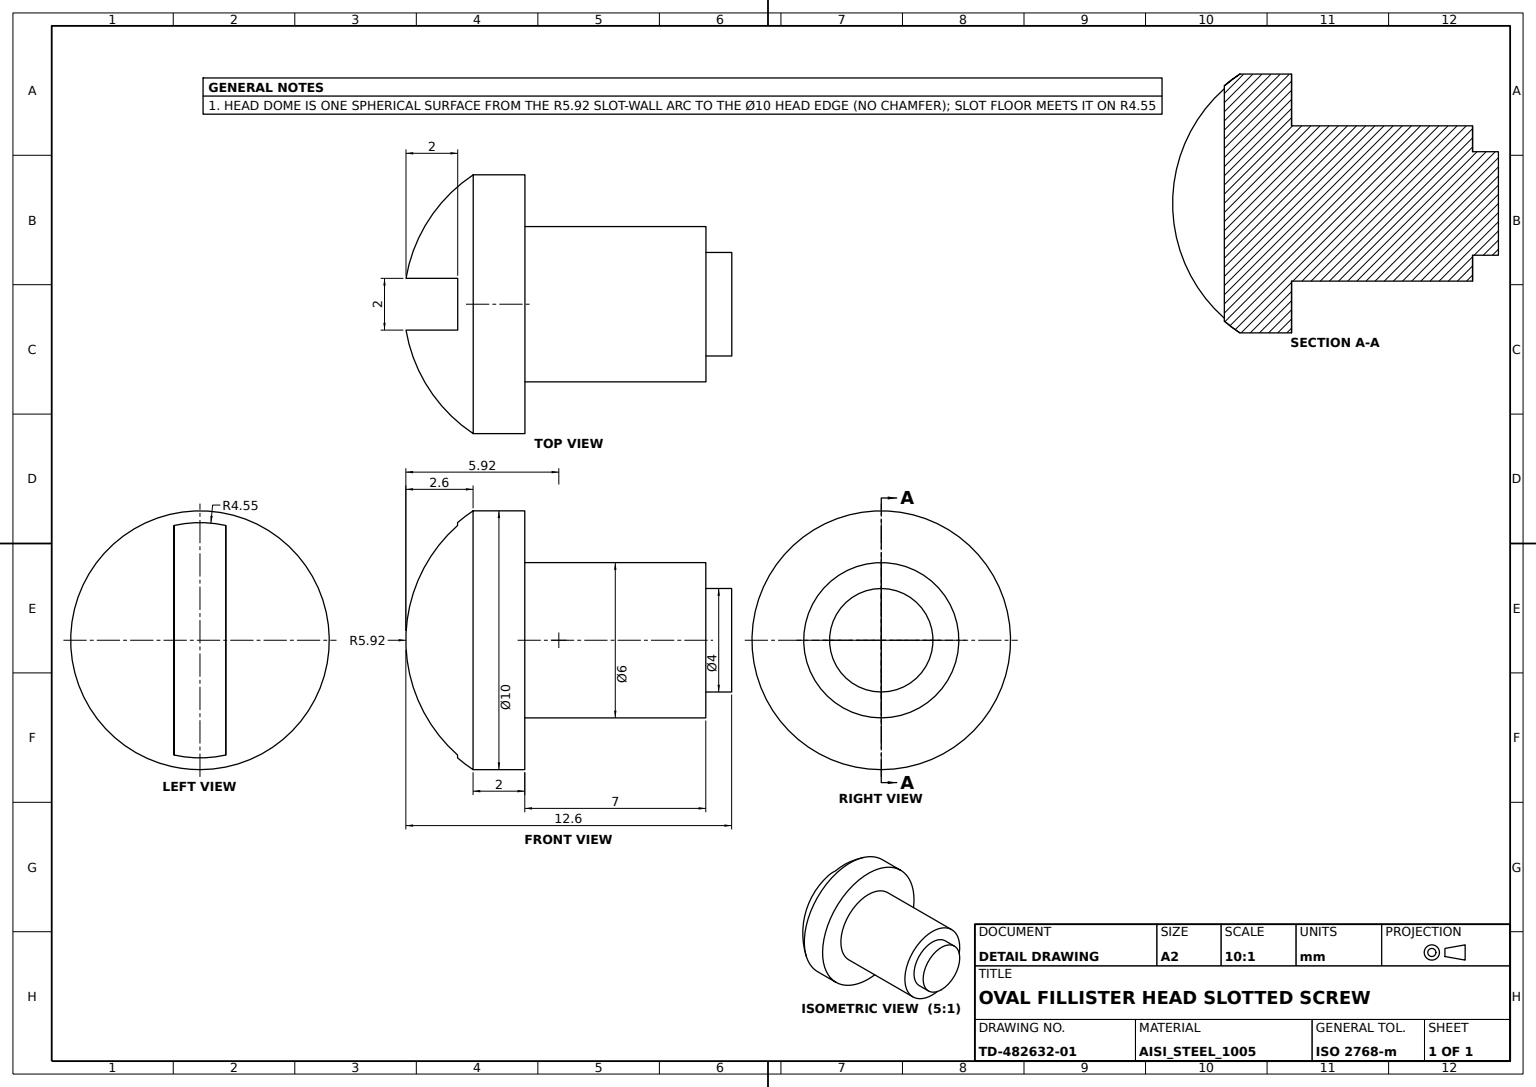
ISO-10303-21;
HEADER;
FILE_DESCRIPTION((''),'2;1');
FILE_NAME('','',(''),(''),'','','');
FILE_SCHEMA(('AUTOMOTIVE_DESIGN'));
ENDSEC;
DATA;
#1=APPLICATION_CONTEXT('');
#2=PRODUCT_CONTEXT('',#1,'mechanical');
#3=PRODUCT('','','',(#2));
#4=PRODUCT_DEFINITION_FORMATION('','',#3);
#5=PRODUCT_DEFINITION_CONTEXT('',#1,'design');
#6=PRODUCT_DEFINITION('','',#4,#5);
#7=PRODUCT_DEFINITION_SHAPE('','',#6);
#8=(LENGTH_UNIT()NAMED_UNIT(*)SI_UNIT(.MILLI.,.METRE.));
#9=(NAMED_UNIT(*)PLANE_ANGLE_UNIT()SI_UNIT($,.RADIAN.));
#10=(NAMED_UNIT(*)SI_UNIT($,.STERADIAN.)SOLID_ANGLE_UNIT());
#11=UNCERTAINTY_MEASURE_WITH_UNIT(LENGTH_MEASURE(0.005),#8,'distance_accuracy_value','');
#12=(GEOMETRIC_REPRESENTATION_CONTEXT(3)GLOBAL_UNCERTAINTY_ASSIGNED_CONTEXT((#11))GLOBAL_UNIT_ASSIGNED_CONTEXT((#8,#9,#10))REPRESENTATION_CONTEXT('',''));
#13=CARTESIAN_POINT('',(0.,0.,-2.));
#14=VERTEX_POINT('',#13);
#15=CARTESIAN_POINT('',(0.,0.,0.));
#16=DIRECTION('',(1.,0.,0.));
#17=DIRECTION('',(0.,0.,-1.));
#18=AXIS2_PLACEMENT_3D('',#15,#16,#17);
#19=CIRCLE('',#18,2.);
#20=EDGE_CURVE('',#14,#14,#19,.T.);
#21=ORIENTED_EDGE('',*,*,#20,.F.);
#22=EDGE_LOOP('',(#21));
#23=FACE_BOUND('',#22,.T.);
#24=CARTESIAN_POINT('',(-1.,0.,-2.));
#25=VERTEX_POINT('',#24);
#26=CARTESIAN_POINT('',(-1.,0.,0.));
#27=AXIS2_PLACEMENT_3D('',#26,#16,#17);
#28=CIRCLE('',#27,2.);
#29=EDGE_CURVE('',#25,#25,#28,.T.);
#30=ORIENTED_EDGE('',*,*,#29,.T.);
#31=EDGE_LOOP('',(#30));
#32=FACE_BOUND('',#31,.T.);
#33=CYLINDRICAL_SURFACE('',#18,2.);
#34=ADVANCED_FACE('',(#23,#32),#33,.T.);
#35=CARTESIAN_POINT('',(-8.,0.,-3.));
#36=VERTEX_POINT('',#35);
#37=CARTESIAN_POINT('',(-8.,0.,0.));
#38=AXIS2_PLACEMENT_3D('',#37,#16,#17);
#39=CIRCLE('',#38,3.);
#40=EDGE_CURVE('',#36,#36,#39,.T.);
#41=ORIENTED_EDGE('',*,*,#40,.T.);
#42=EDGE_LOOP('',(#41));
#43=FACE_BOUND('',#42,.T.);
#44=CARTESIAN_POINT('',(-1.,0.,-3.));
#45=VERTEX_POINT('',#44);
#46=CIRCLE('',#27,3.);
#47=EDGE_CURVE('',#45,#45,#46,.T.);
#48=ORIENTED_EDGE('',*,*,#47,.F.);
#49=EDGE_LOOP('',(#48));
#50=FACE_BOUND('',#49,.T.);
#51=CYLINDRICAL_SURFACE('',#18,3.);
#52=ADVANCED_FACE('',(#43,#50),#51,.T.);
#53=CARTESIAN_POINT('',(-10.,0.,-5.));
#54=VERTEX_POINT('',#53);
#55=CARTESIAN_POINT('',(-10.,0.,0.));
#56=AXIS2_PLACEMENT_3D('',#55,#16,#17);
#57=CIRCLE('',#56,5.);
#58=EDGE_CURVE('',#54,#54,#57,.T.);
#59=ORIENTED_EDGE('',*,*,#58,.F.);
#60=EDGE_LOOP('',(#59));
#61=FACE_BOUND('',#60,.T.);
#62=CARTESIAN_POINT('',(-10.599455,1.,4.434447));
#63=VERTEX_POINT('',#62);
#64=CARTESIAN_POINT('',(-10.599455,-1.,4.434447));
#65=VERTEX_POINT('',#64);
#66=CARTESIAN_POINT('',(-10.599455,0.,0.));
#67=DIRECTION('',(-1.,0.,0.));
#68=DIRECTION('',(0.,0.,1.));
#69=AXIS2_PLACEMENT_3D('',#66,#67,#68);
#70=CIRCLE('',#69,4.545802);
#71=EDGE_CURVE('',#63,#65,#70,.F.);
#72=ORIENTED_EDGE('',*,*,#71,.T.);
#73=CARTESIAN_POINT('',(-10.599455,-1.,-4.434447));
#74=VERTEX_POINT('',#73);
#75=CARTESIAN_POINT('',(-6.683375,-1.,0.));
#76=DIRECTION('',(0.,1.,0.));
#77=AXIS2_PLACEMENT_3D('',#75,#76,#68);
#78=CIRCLE('',#77,5.91608);
#79=EDGE_CURVE('',#65,#74,#78,.F.);
#80=ORIENTED_EDGE('',*,*,#79,.T.);
#81=CARTESIAN_POINT('',(-10.599455,1.,-4.434447));
#82=VERTEX_POINT('',#81);
#83=EDGE_CURVE('',#74,#82,#70,.F.);
#84=ORIENTED_EDGE('',*,*,#83,.T.);
#85=CARTESIAN_POINT('',(-6.683375,1.,0.));
#86=DIRECTION('',(0.,-1.,0.));
#87=AXIS2_PLACEMENT_3D('',#85,#86,#16);
#88=CIRCLE('',#87,5.91608);
#89=EDGE_CURVE('',#82,#63,#88,.F.);
#90=ORIENTED_EDGE('',*,*,#89,.T.);
#91=EDGE_LOOP('',(#72,#80,#84,#90));
#92=FACE_BOUND('',#91,.T.);
#93=CARTESIAN_POINT('',(-6.683375,0.,0.));
#94=AXIS2_PLACEMENT_3D('',#93,#16,#76);
#95=SPHERICAL_SURFACE('',#94,6.);
#96=ADVANCED_FACE('',(#61,#92),#95,.T.);
#97=ORIENTED_EDGE('',*,*,#58,.T.);
#98=EDGE_LOOP('',(#97));
#99=FACE_BOUND('',#98,.T.);
#100=CARTESIAN_POINT('',(-8.,0.,-5.));
#101=VERTEX_POINT('',#100);
#102=CIRCLE('',#38,5.);
#103=EDGE_CURVE('',#101,#101,#102,.T.);
#104=ORIENTED_EDGE('',*,*,#103,.F.);
#105=EDGE_LOOP('',(#104));
#106=FACE_BOUND('',#105,.T.);
#107=CYLINDRICAL_SURFACE('',#18,5.);
#108=ADVANCED_FACE('',(#99,#106),#107,.T.);
#109=ORIENTED_EDGE('',*,*,#89,.F.);
#110=CARTESIAN_POINT('',(-10.599455,1.,7.));
#111=VECTOR('',#17,1000.);
#112=LINE('',#110,#111);
#113=EDGE_CURVE('',#63,#82,#112,.T.);
#114=ORIENTED_EDGE('',*,*,#113,.F.);
#115=EDGE_LOOP('',(#109,#114));
#116=FACE_BOUND('',#115,.T.);
#117=AXIS2_PLACEMENT_3D('',#110,#86,#16);
#118=PLANE('',#117);
#119=ADVANCED_FACE('',(#116),#118,.T.);
#120=ORIENTED_EDGE('',*,*,#20,.T.);
#121=EDGE_LOOP('',(#120));
#122=FACE_BOUND('',#121,.T.);
#123=PLANE('',#18);
#124=ADVANCED_FACE('',(#122),#123,.T.);
#125=ORIENTED_EDGE('',*,*,#79,.F.);
#126=CARTESIAN_POINT('',(-10.599455,-1.,7.));
#127=LINE('',#126,#111);
#128=EDGE_CURVE('',#65,#74,#127,.T.);
#129=ORIENTED_EDGE('',*,*,#128,.T.);
#130=EDGE_LOOP('',(#125,#129));
#131=FACE_BOUND('',#130,.T.);
#132=CARTESIAN_POINT('',(-12.599455,-1.,7.));
#133=AXIS2_PLACEMENT_3D('',#132,#76,#68);
#134=PLANE('',#133);
#135=ADVANCED_FACE('',(#131),#134,.T.);
#136=ORIENTED_EDGE('',*,*,#103,.T.);
#137=EDGE_LOOP('',(#136));
#138=FACE_BOUND('',#137,.T.);
#139=ORIENTED_EDGE('',*,*,#40,.F.);
#140=EDGE_LOOP('',(#139));
#141=FACE_BOUND('',#140,.T.);
#142=CARTESIAN_POINT('',(-8.,3.,0.));
#143=AXIS2_PLACEMENT_3D('',#142,#16,#17);
#144=PLANE('',#143);
#145=ADVANCED_FACE('',(#138,#141),#144,.T.);
#146=ORIENTED_EDGE('',*,*,#83,.F.);
#147=ORIENTED_EDGE('',*,*,#128,.F.);
#148=ORIENTED_EDGE('',*,*,#71,.F.);
#149=ORIENTED_EDGE('',*,*,#113,.T.);
#150=EDGE_LOOP('',(#146,#147,#148,#149));
#151=FACE_BOUND('',#150,.T.);
#152=CARTESIAN_POINT('',(-10.599455,1.,0.));
#153=AXIS2_PLACEMENT_3D('',#152,#67,#68);
#154=PLANE('',#153);
#155=ADVANCED_FACE('',(#151),#154,.T.);
#156=ORIENTED_EDGE('',*,*,#47,.T.);
#157=EDGE_LOOP('',(#156));
#158=FACE_BOUND('',#157,.T.);
#159=ORIENTED_EDGE('',*,*,#29,.F.);
#160=EDGE_LOOP('',(#159));
#161=FACE_BOUND('',#160,.T.);
#162=CARTESIAN_POINT('',(-1.,2.,0.));
#163=AXIS2_PLACEMENT_3D('',#162,#16,#17);
#164=PLANE('',#163);
#165=ADVANCED_FACE('',(#158,#161),#164,.T.);
#166=CLOSED_SHELL('',(#34,#52,#96,#108,#119,#124,#135,#145,#155,#165));
#167=MANIFOLD_SOLID_BREP('',#166);
#168=ADVANCED_BREP_SHAPE_REPRESENTATION('',(#167),#12);
#169=SHAPE_DEFINITION_REPRESENTATION(#7,#168);
ENDSEC;
END-ISO-10303-21;
